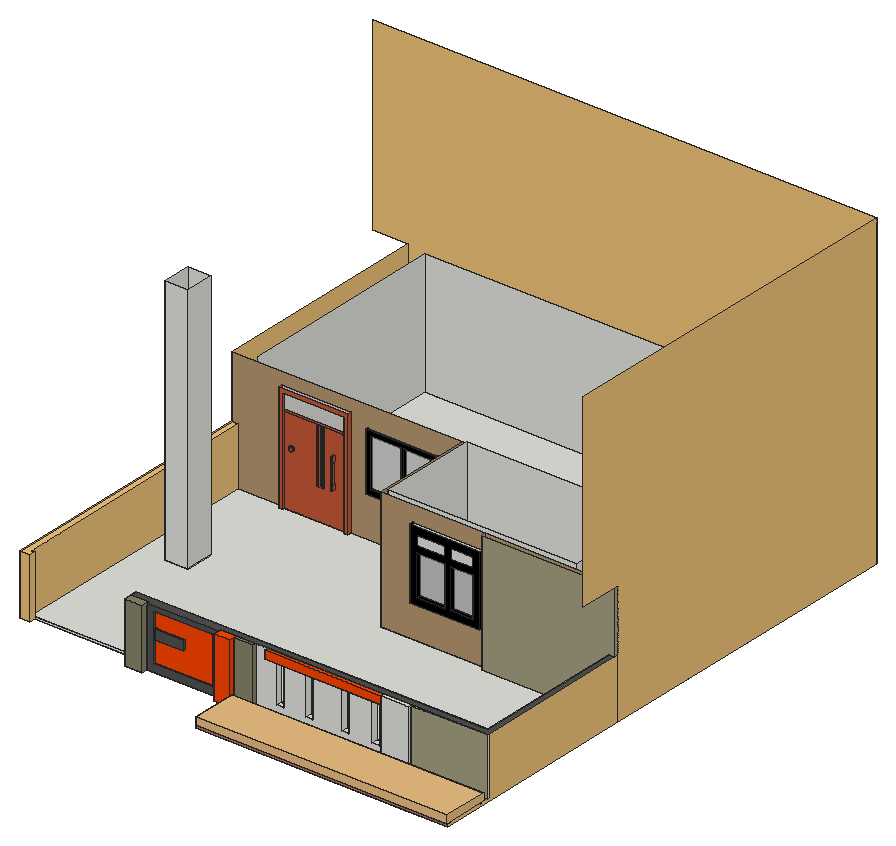
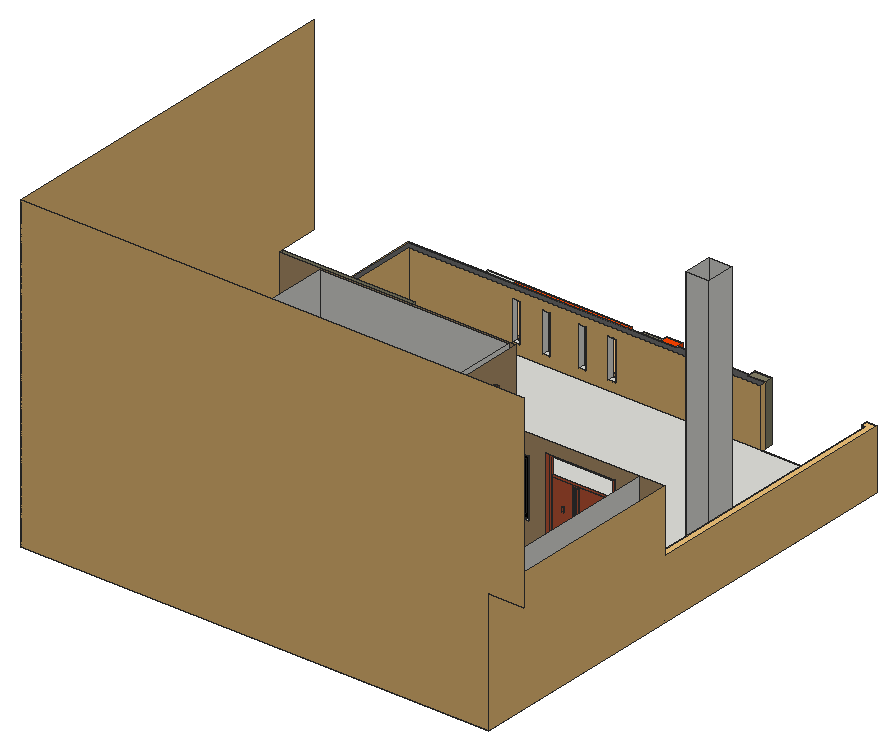
# SketchUp Ruby script. Lengths in inches.
U = 1.inch
M = Sketchup.active_model
def pt(a) = Geom::Point3d.new(a.map { |v| v * U })
def face(e, loops, mat)
  f = e.add_face(loops[0].map { |a| pt(a) })
  loops[1..].each { |l| e.add_face(l.map { |a| pt(a) }).erase! }
  f.material = f.back_material = mat if mat
  f
end
# faces: each face lists its corners as indices into pts; further lists are holes
def faces(e, pts, list, mat = nil) = list.each { |f| face(e, (f[0].is_a?(Array) ? f : [f]).map { |l| l.map { |i| pts[i] } }, mat) }
# xy, xz, yz: faces in a plane at the given z, y or x. An outline is a flat list of corners, or four numbers for a rectangle; further outlines are holes
def ring(l) = l.size == 4 ? [[l[0], l[1]], [l[2], l[1]], [l[2], l[3]], [l[0], l[3]]] : l.each_slice(2).to_a
def flat(e, list, mat, &to3) = list.each { |f| face(e, (f[0].is_a?(Array) ? f : [f]).map { |l| ring(l).map { |u, v| to3.(u, v) } }, mat) }
def xy(e, z, list, mat = nil) = flat(e, list, mat) { |x, y| [x, y, z] }
def xz(e, y, list, mat = nil) = flat(e, list, mat) { |x, z| [x, y, z] }
def yz(e, x, list, mat = nil) = flat(e, list, mat) { |y, z| [x, y, z] }
def lines(e, pts, list) = list.each { |a, b| e.add_line(pt(pts[a]), pt(pts[b])) }
# prism: a flat outline (further loops are holes) pulled along v
def prism(e, loops, v, mat = nil)
  f = face(e, loops, mat); d = Geom::Vector3d.new(v.map { |x| x * U })
  f.pushpull(f.normal.samedirection?(d) ? d.length : -d.length)
end
def box(e, o, s, mat = nil) = prism(e, [[o, [o[0] + s[0], o[1], o[2]], [o[0] + s[0], o[1] + s[1], o[2]], [o[0], o[1] + s[1], o[2]]]], [0, 0, s[2]], mat)
def at(x, y, z, deg = 0) = Geom::Transformation.translation(pt([x, y, z])) * Geom::Transformation.rotation(ORIGIN, Z_AXIS, deg.degrees)
def axes(o, x, y, z) = Geom::Transformation.new([*x, 0, *y, 0, *z, 0, *pt(o).to_a, 1])
def part(name) = M.definitions.add(name)
# library, detail: a bought-in or finely detailed component or shape, given as its bounding box
def library(name, o, s) = part(name).tap { |d| box(d.entities, o, s) }
def detail(e, o, s) = box(e.add_group.entities, o, s)
def put(e, d, t, mat = nil) = e.add_instance(d, t).tap { |i| i.material = mat if mat }
def group(e, t, mat = nil) = e.add_group.tap { |g| g.transformation = t; g.material = mat if mat }.entities
root = M.entities
M.materials.add("[0024_OrangeRed]").color = [255, 69, 0]
M.materials.add("[0036_BurlyWood]").color = [181, 150, 110]
M.materials.add("[0135_DarkGray]").color = [81, 81, 81]
M.materials.add("[0137_Black]").color = [0, 0, 0]
M.materials.add("[Stone Coursed Rough]").color = [165, 160, 130]
M.materials.add("[Stone Coursed Rough]2").color = [135, 131, 106]
M.materials.add("[Stone Flagstone Ashlar]").color = [175, 116, 102]
M.materials.add("[Translucent Glass Gray]").color = [165, 165, 165]
M.materials["[Translucent Glass Gray]"].alpha = 0.5
M.materials.add("[Wood Bamboo]").color = [196, 88, 55]
M.materials.add("[Wood Floor Parquet]").color = [145, 89, 39]
M.materials.add("[Wood OSB]").color = [240, 195, 122]
c1 = library("Untitled.bahçe+çiçek+bitki+zemin+alanları",[0,-19.69,0],[135.94,19.69,5.51])
xy(root,0,[[365.11,0,365.11,74.4375,341.99,74.4375,341.99,71.4375,237.93,71.4375,237.93,74.4375,212.37,74.4375,212.37,83.4375,65.77,83.4375,65.77,74.4375,51.5625,74.4375,51.5625,176.8125,674.75,176.8125,674.75,0],[674.75,0,730.1875,176.8125],[341.99,62.4375,365.11,74.4375],[[51.5625,176.8125,51.5625,457.875,123.72,457.875,123.72,451.875,129.72,451.875,129.72,454.875,217.79,454.875,217.79,451.875,223.79,451.875,223.79,457.875,385.5,457.875,385.5,434.95,379.5,434.95,379.5,429.09,382.5,429.09,382.5,353.72,379.5,353.72,379.5,347.86,385.5,347.86,385.5,309.3125,730.1875,309.3125,730.1875,176.8125],[99.47,277.08,132.15,318.33]],[99.47,277.08,132.15,293.9],
  [99.47,293.9,132.15,297.46],[99.47,297.46,132.15,318.33],[[385.5,309.3125,385.5,457.875,51.5625,457.875,51.5625,776.8125,730.1875,776.8125,730.1875,457.875,391.5,457.875,391.5,315.3125,665.75,315.3125,665.75,309.3125],[83.75,463.875,665.75,767.8125]],[665.75,309.3125,730.1875,457.875],[391.5,315.3125,665.75,457.875],
  [379.5,347.86,385.5,353.72],[382.5,353.72,385.5,429.09],[379.5,429.09,385.5,434.95],[123.72,451.875,129.72,457.875],[217.79,451.875,223.79,457.875],
  [129.72,454.875,217.79,457.875],[83.75,463.875,665.75,767.8125]])
xy(root,0,[[212.37,62.4375,237.93,74.4375]],"[Stone Coursed Rough]2")
xy(root,3,[[[60.5625,83.4375,721.1875,83.4375,721.1875,303.3125,537.22,303.3125,537.22,309.3125,385.5,309.3125,385.5,347.86,379.5,347.86,379.5,353.72,382.5,353.72,382.5,429.09,379.5,429.09,379.5,434.95,385.5,434.95,385.5,457.875,223.79,457.875,223.79,451.875,217.79,451.875,217.79,454.875,129.72,454.875,129.72,451.875,123.72,451.875,123.72,457.875,60.5625,457.875],[99.47,277.08,132.15,318.33]],[665.75,303.3125,674.75,309.3125]])
xy(root,3,[[537.22,303.3125,665.75,309.3125],[674.75,303.3125,721.1875,309.3125]],"[0036_BurlyWood]")
xy(root,4.36,[[578.98,68.3125,619.36,74.4375],[365.11,69.0625,393.43,74.4375],[619.36,72.25,730.1875,74.4375],[380.5,401.85,382.5,413.1]])
xy(root,4.36,[[365.11,0,730.1875,0,730.1875,72.25,619.36,72.25,619.36,68.3125,578.98,68.3125,578.98,74.4375,393.43,74.4375,393.43,69.0625,365.11,69.0625]],"[Stone Flagstone Ashlar]")
xy(root,5.86,[[380.5,370,382.5,379.19]])
xy(root,10.6875,[[247.08,71.4375,333.32,74.4375]],"[0135_DarkGray]")
xy(root,17.02,[[422.58,74.4375,432.83,83.4375],[464.89,74.4375,475.14,83.4375],[516.89,74.4375,527.14,83.4375],[561.58,74.4375,571.83,83.4375]])
xy(root,41.99,[[249.33,71.4375,290.39,74.4375]],"[0135_DarkGray]")
xy(root,49.34,[[178.27,453.875,181.02,454.875],[184.71,453.875,187.46,454.875]],"[Wood Bamboo]")
xy(root,52.45,[[199.87,450.875,203.18,454.875]],"[Wood Bamboo]")
xy(root,53.54,[[432.98,303.3125,534.54,309.3125]],"[0137_Black]")
xy(root,56.18,[[249.33,71.4375,290.39,74.4375]],"[0135_DarkGray]")
xy(root,59.95,[[199.87,450.875,203.18,452.875]])
xy(root,59.95,[[199.87,452.875,203.18,454.875]],"[Wood Bamboo]")
xy(root,63.64,[[247.84,454.875,349.34,457.875]])
xy(root,63.65,[[443.09,303.3125,483.76,309.3125],[492.14,303.3125,524.43,309.3125]],"[0137_Black]")
xy(root,70.35,[[254.5625,454.875,298.59,457.875],[303.24,454.875,342.625,457.875]],"[0137_Black]")
xy(root,72.23,[[380.5,370,382.5,379.19]],"[Wood Floor Parquet]")
xy(root,72.61,[[380.5,401.85,382.5,413.1]],"[Wood Floor Parquet]")
xy(root,74.14,[[422.58,74.4375,432.83,83.4375],[464.89,74.4375,475.14,83.4375],[516.89,74.4375,527.14,83.4375],[561.58,74.4375,571.83,83.4375]])
xy(root,75.4375,[[410.42,69.0625,578.98,74.4375]],"[0024_OrangeRed]")
xy(root,79.34,[[247.08,71.4375,333.32,74.4375]],"[0135_DarkGray]")
xy(root,82.78,[[378.5,375.35,382.5,377.48],[378.5,377.48,380.5,406.16],[378.5,406.16,382.5,408.29]],"[Wood Floor Parquet]")
xy(root,87,[[578.98,68.3125,619.36,74.4375],[619.36,72.25,730.1875,74.4375]])
xy(root,87,[[341.99,62.4375,365.11,74.4375],[410.42,69.0625,578.98,74.4375]],"[0024_OrangeRed]")
xy(root,87,[[721.1875,303.3125,730.1875,309.3125]],"[0036_BurlyWood]")
xy(root,87,[[237.93,71.4375,341.99,71.4375,341.99,74.4375,730.1875,74.4375,730.1875,303.3125,721.1875,303.3125,721.1875,83.4375,212.37,83.4375,212.37,74.4375,237.93,74.4375]],"[0135_DarkGray]")
xy(root,87,[[212.37,62.4375,237.93,74.4375],[365.11,69.0625,393.43,74.4375]],"[Stone Coursed Rough]2")
xy(root,87,[[51.5625,74.4375,65.77,74.4375,65.77,83.4375,60.5625,83.4375,60.5625,457.875,51.5625,457.875]],"[Wood OSB]")
xy(root,87.65,[[378.5,375.35,382.5,377.48],[378.5,377.48,380.5,406.16],[378.5,406.16,382.5,408.29]],"[Wood Floor Parquet]")
xy(root,88.76,[[199.87,450.875,203.18,452.875]])
xy(root,88.76,[[199.87,452.875,203.18,454.875]],"[Wood Bamboo]")
xy(root,95.86,[[380.5,358.84,382.5,422.97]],"[Wood Floor Parquet]")
xy(root,96.26,[[199.87,450.875,203.18,454.875]])
xy(root,121.25,[[443.09,303.3125,483.76,309.3125],[492.14,303.3125,524.43,309.3125]],"[0137_Black]")
xy(root,127.34,[[178.27,453.875,181.02,454.875],[184.71,453.875,187.46,454.875]])
xy(root,129.38,[[129.72,453.875,217.79,454.875]],"[Wood Bamboo]")
xy(root,129.8,[[380.5,358.84,382.5,422.97]],"[Wood Floor Parquet]")
xz(root,0,[[365.11,0,730.1875,4.36]],"[Stone Flagstone Ashlar]")
xz(root,62.4375,[[341.99,0,365.11,87]],"[0024_OrangeRed]")
xz(root,62.4375,[[212.37,0,237.93,87]],"[Stone Coursed Rough]2")
xz(root,68.3125,[[578.98,4.36,619.36,87]])
xz(root,69.0625,[[410.42,75.4375,578.98,87]],"[0024_OrangeRed]")
xz(root,69.0625,[[365.11,4.36,393.43,87]],"[Stone Coursed Rough]2")
xz(root,71.4375,[[[237.93,0,341.99,87],[247.08,10.6875,333.32,79.34]],[249.33,41.99,290.39,56.18]],"[0135_DarkGray]")
xz(root,72.25,[[619.36,4.36,730.1875,87]],"[Stone Coursed Rough]")
xz(root,74.4375,[[212.37,0,237.93,87],[341.99,0,365.11,87],[365.11,4.36,393.43,87],[[393.43,4.36,578.98,4.36,578.98,75.4375,410.42,75.4375,410.42,87,393.43,87],[422.58,17.02,432.83,74.14],[561.58,17.02,571.83,74.14],[516.89,17.02,527.14,74.14],[464.89,17.02,475.14,74.14]],[578.98,4.36,619.36,87],
  [619.36,4.36,730.1875,87],[410.42,75.4375,578.98,87]])
xz(root,74.4375,[[[247.08,10.6875,333.32,79.34],[249.33,41.99,290.39,56.18]]],"[0024_OrangeRed]")
xz(root,74.4375,[[51.5625,0,65.77,87]],"[Wood OSB]")
xz(root,83.4375,[[65.77,0,212.37,3],[60.5625,3,65.77,87]])
xz(root,83.4375,[[[212.37,3,721.1875,87],[422.58,17.02,432.83,74.14],[561.58,17.02,571.83,74.14],[516.89,17.02,527.14,74.14],[464.89,17.02,475.14,74.14]]],"[Wood OSB]")
xz(root,277.08,[[99.47,0,132.15,3],[99.47,3,132.15,366]])
xz(root,303.3125,[[[432.98,53.54,534.54,155.1],[443.09,63.65,483.76,121.25],[492.14,63.65,524.43,121.25],[443.09,130.33,483.76,144.99],[492.14,130.33,524.43,144.99]]],"[0137_Black]")
xz(root,303.3125,[[537.22,3,721.1875,3,721.1875,87,730.1875,87,730.1875,177.375,537.22,177.375]],"[Stone Coursed Rough]")
xz(root,309.3125,[[385.5,0,665.75,3],[665.75,0,674.75,3],[674.75,0,730.1875,3],[721.1875,3,730.1875,87]])
xz(root,309.3125,[[[385.5,3,537.22,177.375],[432.98,53.54,534.54,155.1]],[537.22,3,537.22,177.375,730.1875,177.375,730.1875,87,721.1875,87,721.1875,3]],"[0036_BurlyWood]")
xz(root,309.3125,[[443.09,63.65,483.76,121.25],[492.14,63.65,524.43,121.25]],"[Translucent Glass Gray]")
xz(root,315.3125,[[391.5,0,665.75,180]])
xz(root,318.33,[[99.47,0,132.15,3],[99.47,3,132.15,366]])
xz(root,347.86,[[379.5,0,385.5,3]])
xz(root,347.86,[[379.5,3,385.5,144.3]],"[Wood Floor Parquet]")
xz(root,353.72,[[379.5,0,382.5,3]])
xz(root,353.72,[[379.5,3,382.5,138.4375]],"[Wood Floor Parquet]")
xz(root,358.84,[[380.5,95.86,382.5,129.8]],"[Wood Floor Parquet]")
xz(root,370,[[380.5,5.86,382.5,72.23]],"[Wood Floor Parquet]")
xz(root,375.35,[[378.5,82.78,382.5,87.65]],"[Wood Floor Parquet]")
xz(root,377.48,[[378.5,82.78,380.5,87.65],[380.5,82.78,382.5,87.65]])
xz(root,379.19,[[380.5,5.86,382.5,72.23]],"[Wood Floor Parquet]")
xz(root,401.85,[[380.5,4.36,382.5,72.61]],"[Wood Floor Parquet]")
xz(root,406.16,[[378.5,82.78,380.5,87.65]])
xz(root,406.16,[[380.5,82.78,382.5,87.65]],"[Wood Floor Parquet]")
xz(root,408.29,[[378.5,82.78,382.5,87.65]],"[Wood Floor Parquet]")
xz(root,413.1,[[380.5,4.36,382.5,72.61]],"[Wood Floor Parquet]")
xz(root,422.97,[[380.5,95.86,382.5,129.8]],"[Wood Floor Parquet]")
xz(root,429.09,[[379.5,0,382.5,3]])
xz(root,429.09,[[379.5,3,382.5,138.4375]],"[Wood Floor Parquet]")
xz(root,434.95,[[379.5,0,385.5,3]])
xz(root,434.95,[[379.5,3,385.5,144.3]],"[Wood Floor Parquet]")
xz(root,450.875,[[199.87,52.45,203.18,59.95],[199.87,59.95,203.18,88.76],[199.87,88.76,203.18,96.26]],"[Wood Bamboo]")
xz(root,451.875,[[123.72,0,129.72,3],[217.79,0,223.79,3]])
xz(root,451.875,[[123.72,3,129.72,3,129.72,153.6875,217.79,153.6875,217.79,3,223.79,3,223.79,159.6875,123.72,159.6875]],"[Wood Bamboo]")
xz(root,452.875,[[199.87,59.95,203.18,88.76]])
xz(root,452.875,[[140.66,81.23,141.49,81.34,142.26,81.65,142.92,82.16,143.42,82.82,143.74,83.59,143.85,84.41,143.74,85.24,143.42,86.01,142.92,86.67,142.26,87.17,141.49,87.49,140.66,87.6,139.84,87.49,139.07,87.17,138.41,86.67,137.9,86.01,137.58,85.24,137.47,84.41,137.58,83.59,137.9,82.82,138.41,82.16,139.07,81.65,139.84,81.34]],"[Wood Bamboo]")
xz(root,453.875,[[178.27,49.34,181.02,127.34],[184.71,49.34,187.46,127.34],[129.72,129.38,217.79,132.36]],"[Wood Bamboo]")
xz(root,454.875,[[129.72,0,217.79,3]])
xz(root,454.875,[[[247.84,63.64,349.34,147.14],[254.5625,70.35,298.59,140.42],[303.24,70.35,342.625,140.42]]],"[0137_Black]")
xz(root,454.875,[[[129.72,3,217.79,129.38],[178.27,49.34,181.02,127.34],[184.71,49.34,187.46,127.34],[140.66,81.23,139.84,81.34,139.07,81.65,138.41,82.16,137.9,82.82,137.58,83.59,137.47,84.41,137.58,85.24,137.9,86.01,138.41,86.67,139.07,87.17,139.84,87.49,140.66,87.6,141.49,87.49,142.26,87.17,142.92,86.67,143.42,86.01,143.74,85.24,143.85,84.41,143.74,83.59,143.42,82.82,142.92,82.16,142.26,81.65,141.49,81.34],[199.87,88.76,203.18,96.26],[199.87,52.45,203.18,59.95]]],"[Wood Bamboo]")
xz(root,457.875,[[223.79,0,385.5,3],[391.5,0,665.75,180]])
xz(root,457.875,[[[60.5625,3,123.72,3,123.72,159.6875,223.79,159.6875,223.79,3,385.5,3,385.5,177.375,51.5625,177.375,51.5625,87,60.5625,87],[247.84,63.64,349.34,147.14]]],"[0036_BurlyWood]")
xz(root,457.875,[[254.5625,70.35,298.59,140.42],[303.24,70.35,342.625,140.42]],"[Translucent Glass Gray]")
xz(root,767.8125,[[83.75,0,665.75,180]])
xz(root,776.8125,[[51.5625,0,51.5625,177.375,0,177.375,0,450,730.1875,450,730.1875,0]],"[Wood OSB]")
yz(root,51.5625,[[74.4375,0,74.4375,87,457.875,87,457.875,177.375,776.8125,177.375,776.8125,0]],"[Wood OSB]")
yz(root,60.5625,[[83.4375,3,457.875,87]],"[Wood OSB]")
yz(root,65.77,[[74.4375,0,83.4375,87]],"[Wood OSB]")
yz(root,83.75,[[463.875,0,767.8125,180]])
yz(root,99.47,[[277.08,0,293.9,3],[293.9,0,297.46,3],[297.46,0,318.33,3],[277.08,3,318.33,366]])
yz(root,123.72,[[451.875,0,457.875,3]])
yz(root,123.72,[[451.875,3,457.875,159.6875]],"[Wood Bamboo]")
yz(root,129.72,[[451.875,0,454.875,3]])
yz(root,129.72,[[451.875,3,454.875,3,454.875,129.38,453.875,129.38,453.875,132.36,454.875,132.36,454.875,153.6875,451.875,153.6875]],"[Wood Bamboo]")
yz(root,132.15,[[277.08,0,293.9,3],[293.9,0,297.46,3],[297.46,0,318.33,3],[277.08,3,318.33,366]])
yz(root,178.27,[[453.875,49.34,454.875,127.34]],"[Wood Bamboo]")
yz(root,181.02,[[453.875,49.34,454.875,127.34]],"[Wood Bamboo]")
yz(root,184.71,[[453.875,49.34,454.875,127.34]],"[Wood Bamboo]")
yz(root,187.46,[[453.875,49.34,454.875,127.34]],"[Wood Bamboo]")
yz(root,199.87,[[450.875,52.45,454.875,59.95],[450.875,59.95,452.875,88.76],[450.875,88.76,454.875,96.26]],"[Wood Bamboo]")
yz(root,203.18,[[450.875,52.45,454.875,59.95],[450.875,59.95,452.875,88.76],[450.875,88.76,454.875,96.26]],"[Wood Bamboo]")
yz(root,212.37,[[62.4375,0,74.4375,87]],"[Stone Coursed Rough]2")
yz(root,212.37,[[74.4375,0,83.4375,87]],"[Wood OSB]")
yz(root,217.79,[[451.875,0,454.875,3]])
yz(root,217.79,[[451.875,3,451.875,153.6875,454.875,153.6875,454.875,132.36,453.875,132.36,453.875,129.38,454.875,129.38,454.875,3]],"[Wood Bamboo]")
yz(root,223.79,[[451.875,0,457.875,3]])
yz(root,223.79,[[451.875,3,457.875,159.6875]],"[Wood Bamboo]")
yz(root,237.93,[[71.4375,0,74.4375,87]])
yz(root,237.93,[[62.4375,0,71.4375,87]],"[Stone Coursed Rough]2")
yz(root,247.08,[[71.4375,10.6875,74.4375,79.34]],"[0135_DarkGray]")
yz(root,247.84,[[454.875,63.64,457.875,147.14]],"[0137_Black]")
yz(root,249.33,[[71.4375,41.99,74.4375,56.18]],"[0135_DarkGray]")
yz(root,254.5625,[[454.875,70.35,457.875,140.42]],"[0137_Black]")
yz(root,290.39,[[71.4375,41.99,74.4375,56.18]],"[0135_DarkGray]")
yz(root,298.59,[[454.875,70.35,457.875,140.42]],"[0137_Black]")
yz(root,303.24,[[454.875,70.35,457.875,140.42]],"[0137_Black]")
yz(root,333.32,[[71.4375,10.6875,74.4375,79.34]],"[0135_DarkGray]")
yz(root,341.99,[[71.4375,0,74.4375,87]])
yz(root,341.99,[[62.4375,0,71.4375,87]],"[0024_OrangeRed]")
yz(root,342.625,[[454.875,70.35,457.875,140.42]],"[0137_Black]")
yz(root,349.34,[[454.875,63.64,457.875,147.14]],"[0137_Black]")
yz(root,365.11,[[62.4375,0,74.4375,4.36],[69.0625,4.36,74.4375,87]])
yz(root,365.11,[[62.4375,4.36,69.0625,87]],"[0024_OrangeRed]")
yz(root,365.11,[[0,0,62.4375,4.36]],"[Stone Flagstone Ashlar]")
yz(root,378.5,[[375.35,82.78,377.48,87.65],[377.48,82.78,406.16,87.65],[406.16,82.78,408.29,87.65]],"[Wood Floor Parquet]")
yz(root,379.5,[[347.86,0,353.72,3],[429.09,0,434.95,3]])
yz(root,379.5,[[347.86,3,347.86,144.3,434.95,144.3,434.95,3,429.09,3,429.09,138.4375,353.72,138.4375,353.72,3]],"[Wood Floor Parquet]")
yz(root,380.5,[[377.48,82.78,406.16,87.65]])
yz(root,380.5,[[401.85,4.36,413.1,72.61],[370,5.86,379.19,72.23],[358.84,95.86,422.97,129.8]],"[Wood Floor Parquet]")
yz(root,382.5,[[353.72,0,429.09,3]])
yz(root,382.5,[[[353.72,3,429.09,138.4375],[358.84,95.86,422.97,129.8],[401.85,4.36,413.1,72.61],[370,5.86,379.19,72.23],[406.16,82.78,408.29,87.65],[375.35,82.78,377.48,87.65]]],"[Wood Floor Parquet]")
yz(root,385.5,[[309.3125,0,347.86,3],[434.95,0,457.875,3]])
yz(root,385.5,[[309.3125,3,309.3125,177.375,457.875,177.375,457.875,3,434.95,3,434.95,144.3,347.86,144.3,347.86,3]],"[0036_BurlyWood]")
yz(root,391.5,[[315.3125,0,457.875,180]])
yz(root,393.43,[[69.0625,4.36,74.4375,87]],"[Stone Coursed Rough]2")
yz(root,410.42,[[69.0625,75.4375,74.4375,87]],"[0024_OrangeRed]")
yz(root,422.58,[[74.4375,17.02,83.4375,74.14]])
yz(root,432.83,[[74.4375,17.02,83.4375,74.14]])
yz(root,432.98,[[303.3125,53.54,309.3125,155.1]],"[0137_Black]")
yz(root,443.09,[[303.3125,63.65,309.3125,121.25]],"[0137_Black]")
yz(root,464.89,[[74.4375,17.02,83.4375,74.14]])
yz(root,475.14,[[74.4375,17.02,83.4375,74.14]])
yz(root,483.76,[[303.3125,63.65,309.3125,121.25]],"[0137_Black]")
yz(root,492.14,[[303.3125,63.65,309.3125,121.25]],"[0137_Black]")
yz(root,516.89,[[74.4375,17.02,83.4375,74.14]])
yz(root,524.43,[[303.3125,63.65,309.3125,121.25]],"[0137_Black]")
yz(root,527.14,[[74.4375,17.02,83.4375,74.14]])
yz(root,534.54,[[303.3125,53.54,309.3125,155.1]],"[0137_Black]")
yz(root,537.22,[[303.3125,3,309.3125,177.375]],"[Stone Coursed Rough]")
yz(root,561.58,[[74.4375,17.02,83.4375,74.14]])
yz(root,571.83,[[74.4375,17.02,83.4375,74.14]])
yz(root,578.98,[[68.3125,4.36,74.4375,75.4375],[68.3125,75.4375,69.0625,87],[69.0625,75.4375,74.4375,87]])
yz(root,619.36,[[68.3125,4.36,72.25,87],[72.25,4.36,74.4375,87]])
yz(root,665.75,[[315.3125,0,457.875,112.57],[463.875,0,767.8125,180],[315.3125,112.57,457.875,180]])
yz(root,721.1875,[[303.3125,3,309.3125,87]],"[0036_BurlyWood]")
yz(root,721.1875,[[83.4375,3,303.3125,87]],"[Wood OSB]")
yz(root,730.1875,[[72.25,4.36,74.4375,87]])
yz(root,730.1875,[[303.3125,87,309.3125,177.375]],"[Stone Coursed Rough]")
yz(root,730.1875,[[0,0,309.3125,0,309.3125,87,74.4375,87,74.4375,4.36,0,4.36],[309.3125,0,776.8125,0,776.8125,450,245.125,450,245.125,177.375,309.3125,177.375]],"[Wood OSB]")
p = [[139.84,454.875,81.34],[140.66,454.875,81.23],[140.66,452.875,81.23],[139.84,452.875,81.34],[141.49,454.875,81.34],[141.49,452.875,81.34],
  [139.07,454.875,81.65],[139.07,452.875,81.65],[142.26,454.875,81.65],[142.26,452.875,81.65],[138.41,454.875,82.16],[138.41,452.875,82.16],
  [142.92,454.875,82.16],[142.92,452.875,82.16],[137.9,454.875,82.82],[137.9,452.875,82.82],[143.42,454.875,82.82],[143.42,452.875,82.82],
  [137.58,454.875,83.59],[137.58,452.875,83.59],[143.74,454.875,83.59],[143.74,452.875,83.59],[137.47,454.875,84.41],[137.47,452.875,84.41],
  [143.85,454.875,84.41],[143.85,452.875,84.41],[137.58,454.875,85.24],[137.58,452.875,85.24],[143.74,454.875,85.24],[143.74,452.875,85.24],
  [137.9,454.875,86.01],[137.9,452.875,86.01],[143.42,454.875,86.01],[143.42,452.875,86.01],[138.41,454.875,86.67],[138.41,452.875,86.67],
  [142.92,454.875,86.67],[142.92,452.875,86.67],[139.07,454.875,87.17],[139.07,452.875,87.17],[142.26,454.875,87.17],[142.26,452.875,87.17],
  [139.84,454.875,87.49],[139.84,452.875,87.49],[141.49,454.875,87.49],[141.49,452.875,87.49],[140.66,454.875,87.6],[140.66,452.875,87.6],
  [674.75,176.8125,0],[674.75,176.8125,3],[60.5625,457.875,3],[51.5625,457.875,3]]
faces(root,p,[[0,1,2,3],[1,4,5,2],[6,0,3,7],[4,8,9,5],[10,6,7,11],[8,12,13,9],[14,10,11,15],[12,16,17,13],
  [18,14,15,19],[16,20,21,17],[22,18,19,23],[20,24,25,21],[26,22,23,27],[24,28,29,25],[30,26,27,31],[28,32,33,29],
  [34,30,31,35],[32,36,37,33],[38,34,35,39],[36,40,41,37],[42,38,39,43],[40,44,45,41],[46,42,43,47],[44,46,47,45]],"[Wood Bamboo]")
lines(root,p,[[48,49],[50,51]])
put(root,c1,axes([365.86,64.93,4.36],[2.68,0,0],[0,3.34,0],[0,0,2]))
